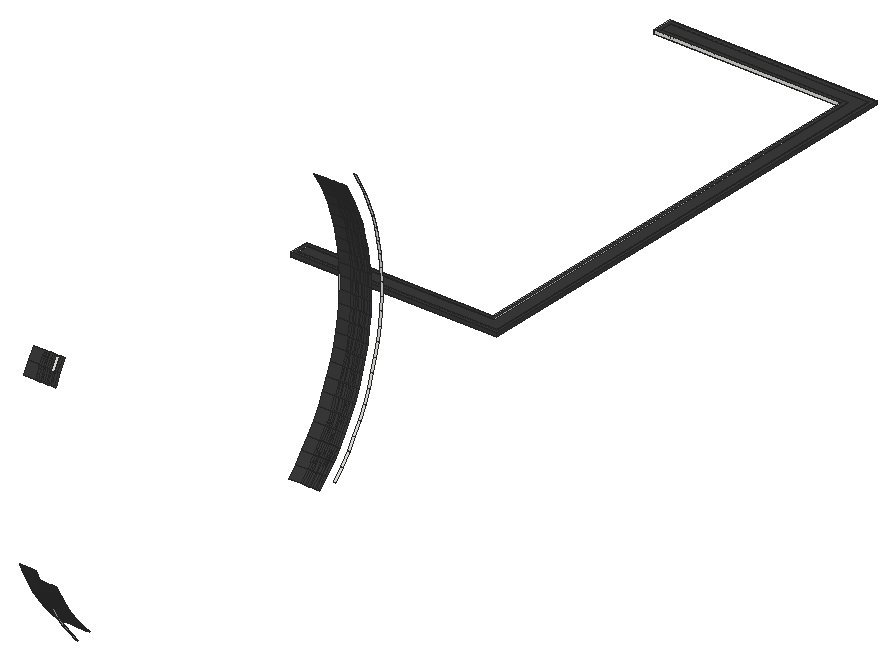
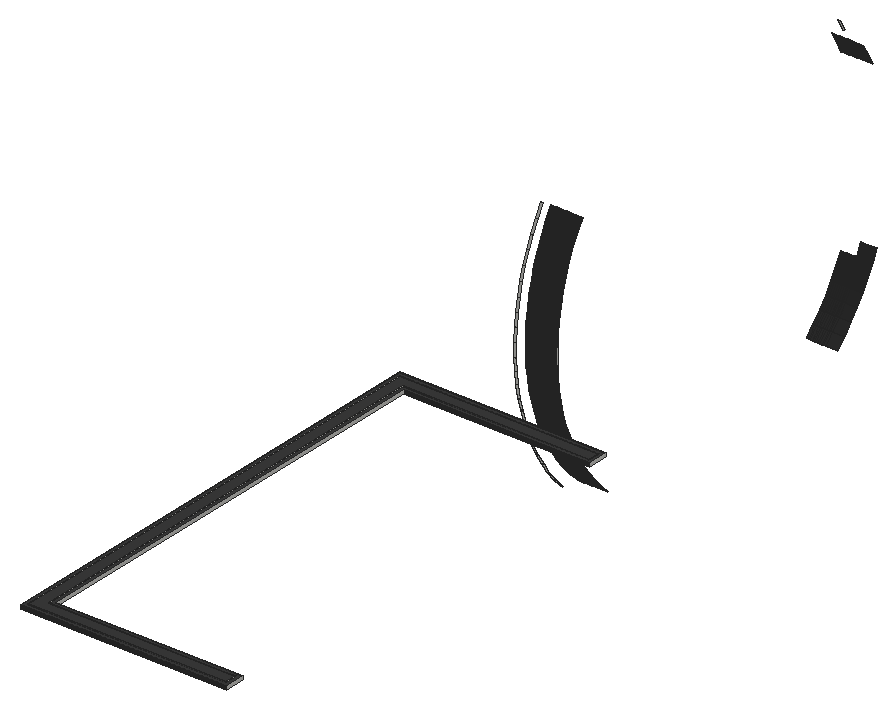
# SketchUp Ruby script. Lengths in inches.
U = 1.inch
M = Sketchup.active_model
def pt(a) = Geom::Point3d.new(a.map { |v| v * U })
def face(e, loops, mat)
  f = e.add_face(loops[0].map { |a| pt(a) })
  loops[1..].each { |l| e.add_face(l.map { |a| pt(a) }).erase! }
  f.material = f.back_material = mat if mat
  f
end
# faces: each face lists its corners as indices into pts; further lists are holes
def faces(e, pts, list, mat = nil) = list.each { |f| face(e, (f[0].is_a?(Array) ? f : [f]).map { |l| l.map { |i| pts[i] } }, mat) }
# xy, xz, yz: faces in a plane at the given z, y or x. An outline is a flat list of corners, or four numbers for a rectangle; further outlines are holes
def ring(l) = l.size == 4 ? [[l[0], l[1]], [l[2], l[1]], [l[2], l[3]], [l[0], l[3]]] : l.each_slice(2).to_a
def flat(e, list, mat, &to3) = list.each { |f| face(e, (f[0].is_a?(Array) ? f : [f]).map { |l| ring(l).map { |u, v| to3.(u, v) } }, mat) }
def xy(e, z, list, mat = nil) = flat(e, list, mat) { |x, y| [x, y, z] }
def xz(e, y, list, mat = nil) = flat(e, list, mat) { |x, z| [x, y, z] }
def yz(e, x, list, mat = nil) = flat(e, list, mat) { |y, z| [x, y, z] }
def lines(e, pts, list) = list.each { |a, b| e.add_line(pt(pts[a]), pt(pts[b])) }
# prism: a flat outline (further loops are holes) pulled along v
def prism(e, loops, v, mat = nil)
  f = face(e, loops, mat); d = Geom::Vector3d.new(v.map { |x| x * U })
  f.pushpull(f.normal.samedirection?(d) ? d.length : -d.length)
end
def box(e, o, s, mat = nil) = prism(e, [[o, [o[0] + s[0], o[1], o[2]], [o[0] + s[0], o[1] + s[1], o[2]], [o[0], o[1] + s[1], o[2]]]], [0, 0, s[2]], mat)
def at(x, y, z, deg = 0) = Geom::Transformation.translation(pt([x, y, z])) * Geom::Transformation.rotation(ORIGIN, Z_AXIS, deg.degrees)
def axes(o, x, y, z) = Geom::Transformation.new([*x, 0, *y, 0, *z, 0, *pt(o).to_a, 1])
def part(name) = M.definitions.add(name)
# library, detail: a bought-in or finely detailed component or shape, given as its bounding box
def library(name, o, s) = part(name).tap { |d| box(d.entities, o, s) }
def detail(e, o, s) = box(e.add_group.entities, o, s)
def put(e, d, t, mat = nil) = e.add_instance(d, t).tap { |i| i.material = mat if mat }
def group(e, t, mat = nil) = e.add_group.tap { |g| g.transformation = t; g.material = mat if mat }.entities
root = M.entities
M.materials.add("[Color M07]").color = [58, 58, 58]
xy(root,286.0625,[[174.13,226.42,174.13,228.68,209.69,228.68,209.69,312.95,174.13,312.95,174.13,315.2,211.95,315.2,211.95,226.42]])
xy(root,286.0625,[[[173.38,225.67,173.38,229.43,208.94,229.43,208.94,312.2,173.38,312.2,173.38,315.95,212.7,315.95,212.7,225.67],[174.13,226.42,211.95,226.42,211.95,315.2,174.13,315.2,174.13,312.95,209.69,312.95,209.69,228.68,174.13,228.68]]],"[Color M07]")
xy(root,286.75,[[[173.38,225.67,212.7,225.67,212.7,315.95,173.38,315.95,173.38,312.2,208.94,312.2,208.94,229.43,173.38,229.43],[174.13,226.42,174.13,228.68,209.69,228.68,209.69,312.95,174.13,312.95,174.13,315.2,211.95,315.2,211.95,226.42]],[174.13,226.42,211.95,226.42,211.95,315.2,174.13,315.2,174.13,312.95,209.69,312.95,209.69,228.68,174.13,228.68]],"[Color M07]")
xz(root,225.67,[[173.38,286.0625,212.7,286.75]],"[Color M07]")
xz(root,226.42,[[174.13,286.0625,211.95,286.75]])
xz(root,228.68,[[174.13,286.0625,176.39,286.75],[176.39,286.0625,209.69,286.75]])
xz(root,229.43,[[173.38,286.0625,176.39,286.75],[176.39,286.0625,208.94,286.75]],"[Color M07]")
xz(root,312.2,[[173.38,286.0625,176.39,286.75],[176.39,286.0625,208.94,286.75]])
xz(root,312.95,[[174.13,286.0625,176.39,286.75],[176.39,286.0625,209.69,286.75]])
xz(root,315.2,[[174.13,286.0625,211.95,286.75]])
xz(root,315.95,[[173.38,286.0625,212.7,286.75]],"[Color M07]")
yz(root,173.38,[[225.67,286.0625,229.43,286.75],[312.2,286.0625,315.95,286.75]])
yz(root,174.13,[[226.42,286.0625,228.68,286.75],[312.95,286.0625,315.2,286.75]])
yz(root,190.96,[[215.22,290.71,215.26,291.31,215.27,293.66,215.22,294.41]])
yz(root,208.94,[[229.43,286.0625,312.2,286.75]])
yz(root,209.69,[[228.68,286.0625,312.95,286.75]])
yz(root,211.95,[[226.42,286.0625,315.2,286.75]])
yz(root,212.7,[[225.67,286.0625,315.95,286.75]],"[Color M07]")
p = [[190.96,146.76,265.83],[193.21,146.76,265.83],[193.21,148.39,264.15],[190.96,148.39,264.15],[193.59,148.39,264.15],[193.59,146.76,265.83],
  [193.96,148.39,264.15],[193.96,146.76,265.83],[194.34,148.39,264.15],[194.34,146.76,265.83],[194.71,148.39,264.15],[194.71,146.76,265.83],
  [195.09,148.39,264.15],[195.09,146.76,265.83],[195.46,148.39,264.15],[195.46,146.76,265.83],[195.84,148.39,264.15],[195.84,146.76,265.83],
  [196.21,148.39,264.15],[196.21,146.76,265.83],[196.59,148.39,264.15],[196.59,146.76,265.83],[196.96,148.39,264.15],[196.96,146.76,265.83],
  [190.96,203.2,264.15],[193.21,203.2,264.15],[193.21,204.84,265.83],[190.96,204.84,265.83],[193.59,204.84,265.83],[193.59,203.2,264.15],
  [193.96,204.84,265.83],[193.96,203.2,264.15],[194.34,204.84,265.83],[194.34,203.2,264.15],[194.71,204.84,265.83],[194.71,203.2,264.15],
  [195.09,204.84,265.83],[195.09,203.2,264.15],[195.46,204.84,265.83],[195.46,203.2,264.15],[195.84,204.84,265.83],[195.84,203.2,264.15],
  [196.21,204.84,265.83],[196.21,203.2,264.15],[196.59,204.84,265.83],[196.59,203.2,264.15],[196.96,204.84,265.83],[196.96,203.2,264.15],
  [196.96,145.08,264.28],[196.96,143.45,266.15],[197.34,143.45,266.15],[197.34,145.08,264.28],[196.96,208.14,266.15],[196.96,206.52,264.28],
  [197.34,206.52,264.28],[197.34,208.14,266.15],[190.96,145.22,267.6],[193.21,145.22,267.6],[193.59,145.22,267.6],[193.96,145.22,267.6],
  [194.34,145.22,267.6],[194.71,145.22,267.6],[195.09,145.22,267.6],[195.46,145.22,267.6],[195.84,145.22,267.6],[196.21,145.22,267.6],
  [196.59,145.22,267.6],[196.96,145.22,267.6],[193.21,206.37,267.6],[190.96,206.37,267.6],[193.59,206.37,267.6],[193.96,206.37,267.6],
  [194.34,206.37,267.6],[194.71,206.37,267.6],[195.09,206.37,267.6],[195.46,206.37,267.6],[195.84,206.37,267.6],[196.21,206.37,267.6],
  [196.59,206.37,267.6],[196.96,206.37,267.6],[196.96,141.94,268.12],[197.34,141.94,268.12],[196.96,209.65,268.12],[197.34,209.65,268.12],
  [190.96,143.79,269.46],[193.21,143.79,269.46],[193.59,143.79,269.46],[193.96,143.79,269.46],[194.34,143.79,269.46],[194.71,143.79,269.46],
  [195.09,143.79,269.46],[195.46,143.79,269.46],[195.84,143.79,269.46],[196.21,143.79,269.46],[196.59,143.79,269.46],[196.96,143.79,269.46],
  [193.21,207.8,269.46],[190.96,207.8,269.46],[193.59,207.8,269.46],[193.96,207.8,269.46],[194.34,207.8,269.46],[194.71,207.8,269.46],
  [195.09,207.8,269.46],[195.46,207.8,269.46],[195.84,207.8,269.46],[196.21,207.8,269.46],[196.59,207.8,269.46],[196.96,207.8,269.46],
  [196.96,140.55,270.17],[197.34,140.55,270.17],[196.96,211.04,270.17],[197.34,211.04,270.17],[190.96,142.48,271.4],[193.21,142.48,271.4],
  [193.59,142.48,271.4],[193.96,142.48,271.4],[194.34,142.48,271.4],[194.71,142.48,271.4],[195.09,142.48,271.4],[195.46,142.48,271.4],
  [195.84,142.48,271.4],[196.21,142.48,271.4],[196.59,142.48,271.4],[196.96,142.48,271.4],[193.21,209.12,271.4],[190.96,209.12,271.4],
  [193.59,209.12,271.4],[193.96,209.12,271.4],[194.34,209.12,271.4],[194.71,209.12,271.4],[195.09,209.12,271.4],[195.46,209.12,271.4],
  [195.84,209.12,271.4],[196.21,209.12,271.4],[196.59,209.12,271.4],[196.96,209.12,271.4],[196.96,139.28,272.3],[197.34,139.28,272.3],
  [196.96,212.3125,272.3],[197.34,212.3125,272.3],[190.96,141.28,273.41],[193.21,141.28,273.41],[193.59,141.28,273.41],[193.96,141.28,273.41],
  [194.34,141.28,273.41],[194.71,141.28,273.41],[195.09,141.28,273.41],[195.46,141.28,273.41],[195.84,141.28,273.41],[196.21,141.28,273.41],
  [196.59,141.28,273.41],[196.96,141.28,273.41],[193.21,210.3125,273.41],[190.96,210.3125,273.41],[193.59,210.3125,273.41],[193.96,210.3125,273.41],
  [194.34,210.3125,273.41],[194.71,210.3125,273.41],[195.09,210.3125,273.41],[195.46,210.3125,273.41],[195.84,210.3125,273.41],[196.21,210.3125,273.41],
  [196.59,210.3125,273.41],[196.96,210.3125,273.41],[196.96,213.45,274.5],[197.34,213.45,274.5],[190.96,140.2,275.49],[193.21,140.2,275.49],
  [193.59,140.2,275.49],[193.96,140.2,275.49],[194.34,140.2,275.49],[194.71,140.2,275.49],[195.09,140.2,275.49],[195.46,140.2,275.49],
  [195.84,140.2,275.49],[196.21,140.2,275.49],[196.59,140.2,275.49],[196.96,140.2,275.49],[193.21,211.39,275.49],[190.96,211.39,275.49],
  [193.59,211.39,275.49],[193.96,211.39,275.49],[194.34,211.39,275.49],[194.71,211.39,275.49],[195.09,211.39,275.49],[195.46,211.39,275.49],
  [195.84,211.39,275.49],[196.21,211.39,275.49],[196.59,211.39,275.49],[196.96,211.39,275.49],[196.96,214.46,276.77],[197.34,214.46,276.77],
  [190.96,139.25,277.63],[193.21,139.25,277.63],[193.59,139.25,277.63],[193.96,139.25,277.63],[193.21,212.34,277.63],[190.96,212.34,277.63],
  [193.59,212.34,277.63],[193.96,212.34,277.63],[194.34,212.34,277.63],[194.71,212.34,277.63],[195.09,212.34,277.63],[195.46,212.34,277.63],
  [195.84,212.34,277.63],[196.21,212.34,277.63],[196.59,212.34,277.63],[196.96,212.34,277.63],[196.96,215.33,279.09],[197.34,215.33,279.09],
  [193.21,213.16,279.83],[190.96,213.16,279.83],[193.59,213.16,279.83],[193.96,213.16,279.83],[194.34,213.16,279.83],[194.71,213.16,279.83],
  [195.09,213.16,279.83],[195.46,213.16,279.83],[195.84,213.16,279.83],[196.21,213.16,279.83],[196.59,213.16,279.83],[196.96,213.16,279.83],
  [196.96,216.06,281.46],[197.34,216.06,281.46],[193.21,213.85,282.07],[190.96,213.85,282.07],[193.59,213.85,282.07],[193.96,213.85,282.07],
  [194.34,213.85,282.07],[194.71,213.85,282.07],[195.09,213.85,282.07],[195.46,213.85,282.07],[195.84,213.85,282.07],[196.21,213.85,282.07],
  [196.59,213.85,282.07],[196.96,213.85,282.07],[196.96,216.65,283.87],[197.34,216.65,283.87],[193.21,214.41,284.34],[190.96,214.41,284.34],
  [193.59,214.41,284.34],[193.96,214.41,284.34],[194.34,214.41,284.34],[194.71,214.41,284.34],[195.09,214.41,284.34],[195.46,214.41,284.34],
  [195.84,214.41,284.34],[196.21,214.41,284.34],[196.59,214.41,284.34],[196.96,214.41,284.34],[196.96,217.09,286.31],[197.34,217.09,286.31],
  [193.21,214.83,286.65],[190.96,214.83,286.65],[193.59,214.83,286.65],[193.96,214.83,286.65],[194.34,214.83,286.65],[194.71,214.83,286.65],
  [195.09,214.83,286.65],[195.46,214.83,286.65],[195.84,214.83,286.65],[196.21,214.83,286.65],[196.59,214.83,286.65],[196.96,214.83,286.65],
  [196.96,217.39,288.77],[197.34,217.39,288.77],[193.21,215.12,288.98],[190.96,215.12,288.98],[193.59,215.12,288.98],[193.96,215.12,288.98],
  [194.34,215.12,288.98],[194.71,215.12,288.98],[195.09,215.12,288.98],[195.46,215.12,288.98],[195.84,215.12,288.98],[196.21,215.12,288.98],
  [196.59,215.12,288.98],[196.96,215.12,288.98],[196.96,217.54,291.24],[197.34,217.54,291.24],[193.21,215.26,291.31],[190.96,215.26,291.31],
  [190.96,215.22,290.71],[193.59,215.26,291.31],[193.96,215.26,291.31],[194.34,215.26,291.31],[194.71,215.26,291.31],[195.09,215.26,291.31],
  [195.46,215.26,291.31],[195.84,215.26,291.31],[196.21,215.26,291.31],[196.59,215.26,291.31],[196.96,215.26,291.31],[196.96,217.55,293.72],
  [197.34,217.55,293.72],[193.21,215.27,293.66],[190.96,215.27,293.66],[193.59,215.27,293.66],[193.96,215.27,293.66],[194.34,215.27,293.66],
  [194.71,215.27,293.66],[195.09,215.27,293.66],[195.46,215.27,293.66],[195.84,215.27,293.66],[196.21,215.27,293.66],[196.59,215.27,293.66],
  [196.96,215.27,293.66],[193.21,215.13,296],[190.96,215.13,296],[190.96,215.22,294.41],[193.59,215.13,296],[193.96,215.13,296],
  [194.34,215.13,296],[194.71,215.13,296],[195.09,215.13,296],[195.46,215.13,296],[195.84,215.13,296],[196.21,215.13,296],
  [196.59,215.13,296],[196.96,215.13,296],[196.96,217.41,296.2],[197.34,217.41,296.2],[193.21,214.86,298.33],[190.96,214.86,298.33],
  [193.59,214.86,298.33],[193.96,214.86,298.33],[194.34,214.86,298.33],[194.71,214.86,298.33],[195.09,214.86,298.33],[195.46,214.86,298.33],
  [195.84,214.86,298.33],[196.21,214.86,298.33],[196.59,214.86,298.33],[196.96,214.86,298.33],[196.96,217.12,298.66],[197.34,217.12,298.66],
  [193.21,214.45,300.63],[190.96,214.45,300.63],[193.59,214.45,300.63],[193.96,214.45,300.63],[194.34,214.45,300.63],[194.71,214.45,300.63],
  [195.09,214.45,300.63],[195.46,214.45,300.63],[195.84,214.45,300.63],[196.21,214.45,300.63],[196.59,214.45,300.63],[196.96,214.45,300.63],
  [196.96,216.69,301.1],[197.34,216.69,301.1],[193.21,213.9,302.91],[190.96,213.9,302.91],[193.59,213.9,302.91],[193.96,213.9,302.91],
  [194.34,213.9,302.91],[194.71,213.9,302.91],[195.09,213.9,302.91],[195.46,213.9,302.91],[195.84,213.9,302.91],[196.21,213.9,302.91],
  [196.59,213.9,302.91],[196.96,213.9,302.91],[196.96,216.11,303.51],[197.34,216.11,303.51],[193.21,213.22,305.15],[190.96,213.22,305.15],
  [193.59,213.22,305.15],[193.96,213.22,305.15],[194.34,213.22,305.15],[194.71,213.22,305.15],[195.09,213.22,305.15],[195.46,213.22,305.15],
  [195.84,213.22,305.15],[196.21,213.22,305.15],[196.59,213.22,305.15],[196.96,213.22,305.15],[196.96,215.39,305.88],[197.34,215.39,305.88],
  [193.21,212.41,307.35],[190.96,212.41,307.35],[193.59,212.41,307.35],[193.96,212.41,307.35],[194.34,212.41,307.35],[194.71,212.41,307.35],
  [195.09,212.41,307.35],[195.46,212.41,307.35],[195.84,212.41,307.35],[196.21,212.41,307.35],[196.59,212.41,307.35],[196.96,212.41,307.35],
  [196.96,214.53,308.21],[197.34,214.53,308.21],[193.21,211.47,309.5],[190.96,211.47,309.5],[193.59,211.47,309.5],[193.96,211.47,309.5],
  [194.34,211.47,309.5],[194.71,211.47,309.5],[195.09,211.47,309.5],[195.46,211.47,309.5],[195.84,211.47,309.5],[196.21,211.47,309.5],
  [196.59,211.47,309.5],[196.96,211.47,309.5],[196.96,213.53,310.48],[197.34,213.53,310.48],[190.96,141.1875,311.59],[193.21,141.1875,311.59],
  [193.21,140.12,309.5],[190.96,140.12,309.5],[193.59,140.12,309.5],[193.59,141.1875,311.59],[193.96,140.12,309.5],[193.96,141.1875,311.59],
  [194.34,140.12,309.5],[194.34,141.1875,311.59],[194.71,140.12,309.5],[194.71,141.1875,311.59],[195.09,140.12,309.5],[195.09,141.1875,311.59],
  [195.46,140.12,309.5],[195.46,141.1875,311.59],[195.84,140.12,309.5],[195.84,141.1875,311.59],[196.21,140.12,309.5],[196.21,141.1875,311.59],
  [196.59,140.12,309.5],[196.59,141.1875,311.59],[196.96,140.12,309.5],[196.96,141.1875,311.59],[193.21,210.4,311.59],[190.96,210.4,311.59],
  [193.59,210.4,311.59],[193.96,210.4,311.59],[194.34,210.4,311.59],[194.71,210.4,311.59],[195.09,210.4,311.59],[195.46,210.4,311.59],
  [195.84,210.4,311.59],[196.21,210.4,311.59],[196.59,210.4,311.59],[196.96,210.4,311.59],[196.96,212.41,312.6875],[197.34,212.41,312.6875],
  [190.96,142.38,313.61],[193.21,142.38,313.61],[193.59,142.38,313.61],[193.96,142.38,313.61],[194.34,142.38,313.61],[194.71,142.38,313.61],
  [195.09,142.38,313.61],[195.46,142.38,313.61],[195.84,142.38,313.61],[196.21,142.38,313.61],[196.59,142.38,313.61],[196.96,142.38,313.61],
  [193.21,209.22,313.61],[190.96,209.22,313.61],[193.59,209.22,313.61],[193.96,209.22,313.61],[194.34,209.22,313.61],[194.71,209.22,313.61],
  [195.09,209.22,313.61],[195.46,209.22,313.61],[195.84,209.22,313.61],[196.21,209.22,313.61],[196.59,209.22,313.61],[196.96,209.22,313.61],
  [196.96,139.1875,312.6875],[196.96,140.44,314.82],[197.34,140.44,314.82],[197.34,139.1875,312.6875],[196.96,211.15,314.82],[197.34,211.15,314.82]]
faces(root,p,[[0,1,2,3],[4,2,1,5],[6,4,5,7],[8,6,7,9],[10,8,9,11],[12,10,11,13],[14,12,13,15],[16,14,15,17],
  [18,16,17,19],[20,18,19,21],[22,20,21,23],[24,25,26,27],[28,26,25,29],[30,28,29,31],[32,30,31,33],[34,32,33,35],
  [36,34,35,37],[38,36,37,39],[40,38,39,41],[42,40,41,43],[44,42,43,45],[46,44,45,47],[56,57,1,0],[5,1,57,58],
  [7,5,58,59],[9,7,59,60],[11,9,60,61],[13,11,61,62],[15,13,62,63],[17,15,63,64],[19,17,64,65],[21,19,65,66],
  [23,21,66,67],[27,26,68,69],[70,68,26,28],[71,70,28,30],[72,71,30,32],[73,72,32,34],[74,73,34,36],[75,74,36,38],
  [76,75,38,40],[77,76,40,42],[78,77,42,44],[79,78,44,46],[84,85,57,56],[58,57,85,86],[59,58,86,87],[60,59,87,88],
  [61,60,88,89],[62,61,89,90],[63,62,90,91],[64,63,91,92],[65,64,92,93],[66,65,93,94],[67,66,94,95],[69,68,96,97],
  [98,96,68,70],[99,98,70,71],[100,99,71,72],[101,100,72,73],[102,101,73,74],[103,102,74,75],[104,103,75,76],[105,104,76,77],
  [106,105,77,78],[107,106,78,79],[112,113,85,84],[86,85,113,114],[87,86,114,115],[88,87,115,116],[89,88,116,117],[90,89,117,118],
  [91,90,118,119],[92,91,119,120],[93,92,120,121],[94,93,121,122],[95,94,122,123],[97,96,124,125],[126,124,96,98],[127,126,98,99],
  [128,127,99,100],[129,128,100,101],[130,129,101,102],[131,130,102,103],[132,131,103,104],[133,132,104,105],[134,133,105,106],[135,134,106,107],
  [140,141,113,112],[114,113,141,142],[115,114,142,143],[116,115,143,144],[117,116,144,145],[118,117,145,146],[119,118,146,147],[120,119,147,148],
  [121,120,148,149],[122,121,149,150],[123,122,150,151],[125,124,152,153],[154,152,124,126],[155,154,126,127],[156,155,127,128],[157,156,128,129],
  [158,157,129,130],[159,158,130,131],[160,159,131,132],[161,160,132,133],[162,161,133,134],[163,162,134,135],[166,167,141,140],[142,141,167,168],
  [143,142,168,169],[144,143,169,170],[145,144,170,171],[146,145,171,172],[147,146,172,173],[148,147,173,174],[149,148,174,175],[150,149,175,176],
  [151,150,176,177],[153,152,178,179],[180,178,152,154],[181,180,154,155],[182,181,155,156],[183,182,156,157],[184,183,157,158],[185,184,158,159],
  [186,185,159,160],[187,186,160,161],[188,187,161,162],[189,188,162,163],[192,193,167,166],[168,167,193,194],[169,168,194,195],[179,178,196,197],
  [198,196,178,180],[199,198,180,181],[200,199,181,182],[201,200,182,183],[202,201,183,184],[203,202,184,185],[204,203,185,186],[205,204,186,187],
  [206,205,187,188],[207,206,188,189],[197,196,210,211],[212,210,196,198],[213,212,198,199],[214,213,199,200],[215,214,200,201],[216,215,201,202],
  [217,216,202,203],[218,217,203,204],[219,218,204,205],[220,219,205,206],[221,220,206,207],[211,210,224,225],[226,224,210,212],[227,226,212,213],
  [228,227,213,214],[229,228,214,215],[230,229,215,216],[231,230,216,217],[232,231,217,218],[233,232,218,219],[234,233,219,220],[235,234,220,221],
  [225,224,238,239],[240,238,224,226],[241,240,226,227],[242,241,227,228],[243,242,228,229],[244,243,229,230],[245,244,230,231],[246,245,231,232],
  [247,246,232,233],[248,247,233,234],[249,248,234,235],[239,238,252,253],[254,252,238,240],[255,254,240,241],[256,255,241,242],[257,256,242,243],
  [258,257,243,244],[259,258,244,245],[260,259,245,246],[261,260,246,247],[262,261,247,248],[263,262,248,249],[253,252,266,267],[268,266,252,254],
  [269,268,254,255],[270,269,255,256],[271,270,256,257],[272,271,257,258],[273,272,258,259],[274,273,259,260],[275,274,260,261],[276,275,261,262],
  [277,276,262,263],[267,266,280,281,282],[283,280,266,268],[284,283,268,269],[285,284,269,270],[286,285,270,271],[287,286,271,272],[288,287,272,273],
  [289,288,273,274],[290,289,274,275],[291,290,275,276],[292,291,276,277],[281,280,295,296],[297,295,280,283],[298,297,283,284],[299,298,284,285],
  [300,299,285,286],[301,300,286,287],[302,301,287,288],[303,302,288,289],[304,303,289,290],[305,304,290,291],[306,305,291,292],[296,295,307,308,309],
  [310,307,295,297],[311,310,297,298],[312,311,298,299],[313,312,299,300],[314,313,300,301],[315,314,301,302],[316,315,302,303],[317,316,303,304],
  [318,317,304,305],[319,318,305,306],[308,307,322,323],[324,322,307,310],[325,324,310,311],[326,325,311,312],[327,326,312,313],[328,327,313,314],
  [329,328,314,315],[330,329,315,316],[331,330,316,317],[332,331,317,318],[333,332,318,319],[323,322,336,337],[338,336,322,324],[339,338,324,325],
  [340,339,325,326],[341,340,326,327],[342,341,327,328],[343,342,328,329],[344,343,329,330],[345,344,330,331],[346,345,331,332],[347,346,332,333],
  [337,336,350,351],[352,350,336,338],[353,352,338,339],[354,353,339,340],[355,354,340,341],[356,355,341,342],[357,356,342,343],[358,357,343,344],
  [359,358,344,345],[360,359,345,346],[361,360,346,347],[351,350,364,365],[366,364,350,352],[367,366,352,353],[368,367,353,354],[369,368,354,355],
  [370,369,355,356],[371,370,356,357],[372,371,357,358],[373,372,358,359],[374,373,359,360],[375,374,360,361],[365,364,378,379],[380,378,364,366],
  [381,380,366,367],[382,381,367,368],[383,382,368,369],[384,383,369,370],[385,384,370,371],[386,385,371,372],[387,386,372,373],[388,387,373,374],
  [389,388,374,375],[379,378,392,393],[394,392,378,380],[395,394,380,381],[396,395,381,382],[397,396,382,383],[398,397,383,384],[399,398,384,385],
  [400,399,385,386],[401,400,386,387],[402,401,387,388],[403,402,388,389],[406,407,408,409],[410,408,407,411],[412,410,411,413],[414,412,413,415],
  [416,414,415,417],[418,416,417,419],[420,418,419,421],[422,420,421,423],[424,422,423,425],[426,424,425,427],[428,426,427,429],[393,392,430,431],
  [432,430,392,394],[433,432,394,395],[434,433,395,396],[435,434,396,397],[436,435,397,398],[437,436,398,399],[438,437,399,400],[439,438,400,401],
  [440,439,401,402],[441,440,402,403],[444,445,407,406],[411,407,445,446],[413,411,446,447],[415,413,447,448],[417,415,448,449],[419,417,449,450],
  [421,419,450,451],[423,421,451,452],[425,423,452,453],[427,425,453,454],[429,427,454,455],[431,430,456,457],[458,456,430,432],[459,458,432,433],
  [460,459,433,434],[461,460,434,435],[462,461,435,436],[463,462,436,437],[464,463,437,438],[465,464,438,439],[466,465,439,440],[467,466,440,441]],"[Color M07]")
faces(root,p,[[48,49,50,51],[52,53,54,55],[49,80,81,50],[82,52,55,83],[80,108,109,81],[110,82,83,111],[108,136,137,109],[138,110,111,139],
  [164,138,139,165],[190,164,165,191],[208,190,191,209],[222,208,209,223],[236,222,223,237],[250,236,237,251],[264,250,251,265],[278,264,265,279],
  [293,278,279,294],[320,293,294,321],[334,320,321,335],[348,334,335,349],[362,348,349,363],[376,362,363,377],[390,376,377,391],[404,390,391,405],
  [442,404,405,443],[468,469,470,471],[472,442,443,473]])
